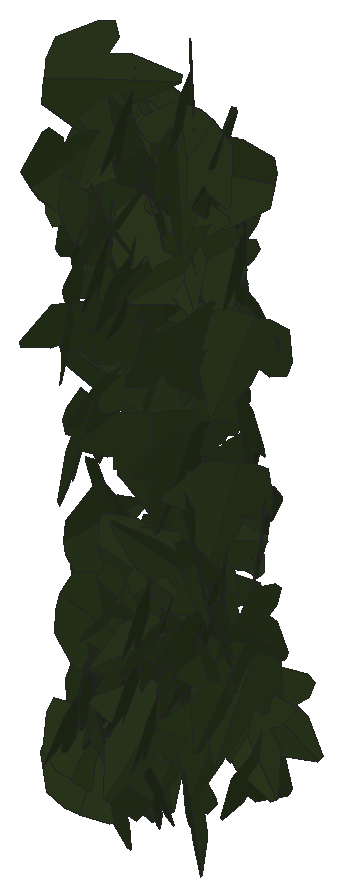
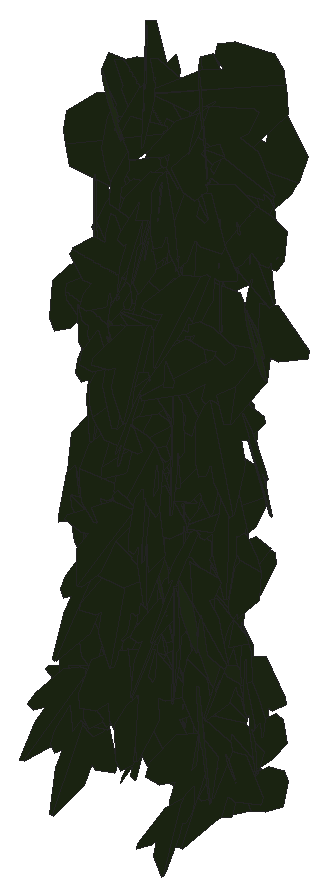
# SketchUp Ruby script. Lengths in inches.
U = 1.inch
M = Sketchup.active_model
def pt(a) = Geom::Point3d.new(a.map { |v| v * U })
def face(e, loops, mat)
  f = e.add_face(loops[0].map { |a| pt(a) })
  loops[1..].each { |l| e.add_face(l.map { |a| pt(a) }).erase! }
  f.material = f.back_material = mat if mat
  f
end
# faces: each face lists its corners as indices into pts; further lists are holes
def faces(e, pts, list, mat = nil) = list.each { |f| face(e, (f[0].is_a?(Array) ? f : [f]).map { |l| l.map { |i| pts[i] } }, mat) }
# xy, xz, yz: faces in a plane at the given z, y or x. An outline is a flat list of corners, or four numbers for a rectangle; further outlines are holes
def ring(l) = l.size == 4 ? [[l[0], l[1]], [l[2], l[1]], [l[2], l[3]], [l[0], l[3]]] : l.each_slice(2).to_a
def flat(e, list, mat, &to3) = list.each { |f| face(e, (f[0].is_a?(Array) ? f : [f]).map { |l| ring(l).map { |u, v| to3.(u, v) } }, mat) }
def xy(e, z, list, mat = nil) = flat(e, list, mat) { |x, y| [x, y, z] }
def xz(e, y, list, mat = nil) = flat(e, list, mat) { |x, z| [x, y, z] }
def yz(e, x, list, mat = nil) = flat(e, list, mat) { |y, z| [x, y, z] }
def lines(e, pts, list) = list.each { |a, b| e.add_line(pt(pts[a]), pt(pts[b])) }
# prism: a flat outline (further loops are holes) pulled along v
def prism(e, loops, v, mat = nil)
  f = face(e, loops, mat); d = Geom::Vector3d.new(v.map { |x| x * U })
  f.pushpull(f.normal.samedirection?(d) ? d.length : -d.length)
end
def box(e, o, s, mat = nil) = prism(e, [[o, [o[0] + s[0], o[1], o[2]], [o[0] + s[0], o[1] + s[1], o[2]], [o[0], o[1] + s[1], o[2]]]], [0, 0, s[2]], mat)
def at(x, y, z, deg = 0) = Geom::Transformation.translation(pt([x, y, z])) * Geom::Transformation.rotation(ORIGIN, Z_AXIS, deg.degrees)
def axes(o, x, y, z) = Geom::Transformation.new([*x, 0, *y, 0, *z, 0, *pt(o).to_a, 1])
def part(name) = M.definitions.add(name)
# library, detail: a bought-in or finely detailed component or shape, given as its bounding box
def library(name, o, s) = part(name).tap { |d| box(d.entities, o, s) }
def detail(e, o, s) = box(e.add_group.entities, o, s)
def put(e, d, t, mat = nil) = e.add_instance(d, t).tap { |i| i.material = mat if mat }
def group(e, t, mat = nil) = e.add_group.tap { |g| g.transformation = t; g.material = mat if mat }.entities
root = M.entities
M.materials.add("efeu2").color = [43, 57, 29]
c1 = part("ivyleaf_10")
p = [[0,0.5,-0.03],[-0.0625,2.02,-0.43],[-0.19,2.01,-0.46],[-0.54,1.05,-0.29],[-0.52,0.625,-0.18],[-0.83,0.76,-0.28],
  [-1.16,0.64,-0.33],[-1.15,0.33,-0.24],[-0.77,-0.39,0.02],[-0.3,-0.51,0.16],[0.04,-0.48,0.23],[-0.02,2.01,-0.4375],
  [-0.06,2.01,-0.43],[0.04,-0.49,0.23],[0.67,-0.49,0.14],[1.38,0.36,-0.2],[1.375,0.51,-0.24],[0.81,0.65,-0.19],
  [0.62,0.59,-0.15],[0.6,1.09,-0.28],[0.5,1.23,-0.31]]
faces(c1.entities,p,[[0,1,2,3,4,5,6,7,8,9,10],[11,12,0,13,14,15,16,17,18,19,20]],"efeu2")
put(root,c1,axes([506.9,136.79,173.25],[0.14298,-0.57574,-0.30284],[-0.08063,0.292,-0.59319],[0.64552,0.164,-0.00701]))
put(root,c1,axes([507.25,136.87,180.96],[-0.48159,0.04123,0.55153],[-0.55018,0.03894,-0.48332],[-0.05645,-0.73116,0.00536]))
put(root,c1,axes([506.58,137.23,179.57],[0.28434,-0.41575,0.47022],[0.3227,-0.34593,-0.501],[0.53835,0.42695,0.05196]))
put(root,c1,axes([506.88,137.7,177.9],[0.03406,-0.68562,-0.00532],[-0.00302,0.00518,-0.68646],[0.68563,0.03408,-0.00276]))
put(root,c1,axes([506.67,137.17,172.16],[0.25361,0.41099,-0.45403],[0.22987,0.38118,0.49226],[0.60538,-0.31691,0.00328]))
put(root,c1,axes([506.84,137.01,177.54],[0.4432,-0.50153,-0.03424],[-0.0221,0.0258,-0.67395],[0.54237,0.41088,0.00052]))
put(root,c1,axes([506.89,137.09,179.24],[-0.46172,-0.52625,-0.10401],[0.07279,0.0745,-0.70007],[0.53147,-0.46739,0.00552]))
put(root,c1,axes([507.1,137.3,176.33],[-0.55796,0.2577,0.27413],[-0.26708,0.07405,-0.61323],[-0.26499,-0.61724,0.04088]))
put(root,c1,axes([506.98,137.88,173.2],[0.21629,-0.56569,-0.2598],[-0.08303,0.24636,-0.60555],[0.61694,0.23148,0.00958]))
put(root,c1,axes([506.71,136.54,181.61],[-0.09839,-0.31052,0.53966],[0.14335,0.5017,0.33646],[-0.63717,0.16082,-0.00764]))
put(root,c1,axes([506.73,137.27,171.58],[0.59865,0.26422,-0.18769],[0.17611,0.07732,0.63862],[0.29733,-0.57779,-0.00037]))
put(root,c1,axes([506.84,138.72,171.91],[-0.02473,0.55753,-0.00621],[0.00369,-0.00584,-0.58031],[-0.60216,-0.02293,-0.0033]))
put(root,c1,axes([506.58,137.39,181.29],[0.5485,0.17555,0.41224],[0.36114,0.21247,-0.571],[-0.2652,0.65242,0.07504]))
put(root,c1,axes([507.17,136.57,180.82],[0.24842,-0.09066,0.51979],[-0.34502,0.40074,0.22851],[-0.42651,-0.37698,0.11791]))
put(root,c1,axes([507.09,136.9375,173.84],[0.05979,-0.2875,-0.63142],[-0.0329,0.63188,-0.29083],[0.69302,0.0548,0.04067]))
put(root,c1,axes([507.38,137.47,182.34],[-0.27318,-0.29829,0.51186],[-0.35183,-0.36898,-0.40669],[0.51239,-0.41239,-0.00635]))
put(root,c1,axes([507.08,137.7,172.24],[-0.609,-0.27487,-0.13611],[0.12561,0.05254,-0.66815],[0.27983,-0.62181,0.00371]))
put(root,c1,axes([507.03,138.19,180.26],[0.03283,0.53443,0.24861],[0.00153,0.2393,-0.55658],[-0.63229,0.02833,0.01156]))
put(root,c1,axes([506.68,137.18,173.43],[0.29168,-0.18018,0.59082],[0.56331,-0.19048,-0.33618],[0.25342,0.63077,0.06725]))
put(root,c1,axes([507.02,137.0625,181.28],[-0.66421,-0.04385,-0.21378],[0.22186,0.009,-0.64121],[0.048,-0.64839,0.00556]))
put(root,c1,axes([507.1,136.64,181.57],[-0.02237,0.43314,0.45119],[-0.07644,0.4295,-0.44947],[-0.65766,-0.06465,0.0369]))
put(root,c1,axes([506.93,137.43,179.04],[0.15008,0.12887,0.69477],[0.1279,0.69359,-0.15627],[-0.69495,0.15547,0.12128]))
put(root,c1,axes([507.14,137.45,174.3125],[0.15323,-0.55835,0.32624],[0.08521,-0.31492,-0.57899],[0.64103,0.17532,-0.00102]))
put(root,c1,axes([507.19,138.24,174.93],[0.32095,-0.51181,-0.2376],[0.00169,0.27421,-0.5884],[0.56427,0.29029,0.13691]))
put(root,c1,axes([507.17,137.69,173.66],[0.08189,-0.52853,0.43053],[0.08188,-0.42286,-0.53469],[0.67675,0.11512,0.0126]))
put(root,c1,axes([507.61,137.62,174.82],[-0.38669,-0.02044,0.48346],[-0.5014,-0.02372,-0.37297],[0.03377,-0.58629,-0.00177]))
put(root,c1,axes([507.36,137.71,180.73],[-0.67386,0.01628,0.13224],[-0.13231,-0.00125,-0.67404],[-0.01573,-0.68671,0.00436]))
put(root,c1,axes([507.31,136.95,180.6],[0.18928,-0.53998,-0.39955],[-0.08333,0.39303,-0.57065],[0.66654,0.20248,0.04212]))
put(root,c1,axes([507.12,137.76,179.85],[-0.53879,-0.3581,-0.20826],[0.22409,0.03542,-0.64065],[0.34841,-0.57655,0.08999]))
put(root,c1,axes([507.17,136.64,176.05],[0.02579,-0.06365,0.59985],[-0.05409,0.57489,0.06813],[-0.62436,-0.05244,0.01887]))
put(root,c1,axes([507.14,136.55,174.95],[-0.00618,0.43263,0.48163],[-0.02651,0.46263,-0.44978],[-0.68393,-0.02184,0.01308]))
put(root,c1,axes([506.82,136.83,183.15],[-0.07026,-0.02384,-0.72695],[0.65355,0.31847,-0.07361],[0.31922,-0.65725,-0.0093]))
put(root,c1,axes([507.53,137.45,174.31],[-0.59782,-0.14347,0.15385],[-0.15413,-0.03901,-0.5947],[0.16057,-0.57163,0.00197]))
put(root,c1,axes([506.89,137.1,175.3125],[-0.09933,0.04464,-0.68674],[0.56951,-0.38419,-0.10734],[-0.38634,-0.57782,0.01832]))
put(root,c1,axes([507.44,137.95,177.9],[0.37613,-0.4555,-0.31889],[-0.04582,0.3583,-0.56583],[0.55414,0.3388,0.16967]))
put(root,c1,axes([507.52,137.35,182.45],[0.38884,0.29811,-0.35452],[-0.28376,-0.21719,-0.48613],[-0.39834,0.44571,0.00023]))
put(root,c1,axes([507.57,137.73,180.09],[-0.439,-0.49286,0.16997],[-0.02017,-0.20599,-0.64937],[0.52095,-0.4233,0.1181]))
put(root,c1,axes([507.375,137.74,174.93],[0.23268,-0.47713,0.31676],[0.15414,-0.26957,-0.54418],[0.59158,0.2579,0.0172]))
put(root,c1,axes([507.43,137.34,180.02],[0.07021,0.57173,0.44951],[-0.03773,0.45386,-0.57136],[-0.7263,0.03168,0.07314]))
put(root,c1,axes([507.09,137.77,178.98],[0.41379,0.00326,-0.54265],[0.50595,0.2444,0.38728],[0.19619,-0.63715,0.14577]))
put(root,c1,axes([507.03,137.42,171.875],[0.10377,-0.08511,-0.7135],[0.54321,-0.46261,0.13418],[-0.47037,-0.55302,-0.00244]))
put(root,c1,axes([507.48,137.55,175.43],[0.11447,-0.4952,-0.43868],[0.13951,0.45325,-0.47525],[0.64668,-0.01013,0.18017]))
put(root,c1,axes([507.71,137.37,172.31],[-0.51777,0.36658,0.27419],[-0.22529,0.1563,-0.6344],[-0.39851,-0.56466,0.0024]))
put(root,c1,axes([507.46,137.57,182.59],[0.09528,0.54935,0.01156],[-0.00154,0.01149,-0.57863],[-0.59341,0.08818,0.00336]))
put(root,c1,axes([507.63,137.33,179.99],[0.18603,-0.63952,-0.18734],[-0.05193,0.17999,-0.66603],[0.66436,0.19314,0.0004]))
put(root,c1,axes([507.41,137.4,177.05],[-0.46287,0.22473,-0.30946],[0.28739,-0.13324,-0.50327],[-0.28212,-0.50445,-0.00494]))
put(root,c1,axes([507.67,137.42,180.86],[-0.21695,-0.64043,-0.11482],[0.06907,0.09768,-0.67535],[0.64697,-0.22518,0.0336]))
put(root,c1,axes([507.66,138.09,174.6],[-0.17825,0.49977,0.26514],[-0.09342,0.2399,-0.54733],[-0.59867,-0.18624,0.00647]))
put(root,c1,axes([508.05,136.78,182.37],[-0.42142,0.09736,0.48472],[-0.50039,0.06123,-0.41672],[-0.11851,-0.60476,0.03584]))
put(root,c1,axes([507.72,136.91,182.95],[0.25353,-0.61713,-0.25077],[-0.04077,0.25344,-0.66492],[0.66488,0.25086,0.05485]))
put(root,c1,axes([507.64,137.68,181.33],[-0.67868,-0.06143,-0.11158],[0.11154,0.00544,-0.68144],[0.0615,-0.68777,0.00458]))
put(root,c1,axes([507.75,137.64,181.38],[0.03236,-0.68955,-0.00584],[-0.00999,0.00537,-0.69024],[0.6895,0.03244,-0.00972]))
put(root,c1,axes([508.13,137.32,181.83],[-0.27876,0.03467,0.53386],[-0.54992,0.06513,-0.27084],[-0.07968,-0.57087,0.00152]))
put(root,c1,axes([507.77,136.92,180.42],[0.02069,-0.57405,-0.40253],[0.01707,0.403,-0.57384],[0.70091,0.00713,0.02586]))
put(root,c1,axes([507.8,137.4375,178.23],[0.40243,0.42699,-0.23491],[-0.24978,-0.09274,-0.57913],[-0.45801,0.42575,0.10944]))
put(root,c1,axes([507.81,137.29,179.79],[-0.18125,-0.6679,0.0763],[-0.00602,-0.07741,-0.6919],[0.67222,-0.18077,0.01438]))
put(root,c1,axes([507.82,136.97,174.01],[0.21995,-0.58813,-0.24273],[-0.04493,0.24183,-0.62666],[0.63467,0.22095,0.03976]))
put(root,c1,axes([507.32,136.96,175.77],[-0.18678,-0.01314,-0.5707],[0.579,-0.12751,-0.17255],[-0.12722,-0.56105,0.05258]))
put(root,c1,axes([507.75,138.41,179.25],[0.11452,0.53998,0.18204],[-0.10046,0.19218,-0.558],[-0.60477,0.07032,0.12716]))
put(root,c1,axes([507.83,138.1,176.28],[0.06611,-0.62024,-0.20868],[0.00551,0.21026,-0.6232],[0.65438,0.0609,0.02633]))
put(root,c1,axes([507.89,138.09,172.87],[-0.22657,-0.5453,0.26649],[0.02259,-0.29184,-0.57795],[0.60651,-0.19284,0.12108]))
put(root,c1,axes([507.91,138.16,180.43],[-0.40528,0.45057,0.0565],[0.03412,-0.04439,0.60982],[0.48896,0.37657,0.00428]))
put(root,c1,axes([507.79,138.54,178.29],[-0.28382,0.49292,-0.09531],[0.04123,-0.08349,-0.58092],[-0.53991,-0.2655,0.00574]))
put(root,c1,axes([508.01,137.24,173.29],[-0.31999,-0.44489,0.41652],[-0.0211,-0.46207,-0.50976],[0.60907,-0.24974,0.20117]))
put(root,c1,axes([508.04,137.07,177.84],[-0.53452,-0.51019,0.01267],[-0.00802,-0.00995,-0.73892],[0.51028,-0.53457,0.00167]))
put(root,c1,axes([508.03,137.46,180.23],[-0.14531,-0.67577,-0.0284],[-0.00877,0.03093,-0.69105],[0.67631,-0.14479,-0.01506]))
put(root,c1,axes([508.01,138.37,179.05],[-0.62141,-0.05793,-0.00008],[0.00008,0.00002,-0.60142],[0.06256,-0.57538,-0.00002]))
put(root,c1,axes([508.03,137.65,178.8125],[0.00198,-0.66951,0.11793],[-0.00178,-0.11793,-0.66951],[0.67981,0.00164,-0.0021]))
put(root,c1,axes([508.33,138.47,178.01],[-0.3906,0.16269,-0.41881],[-0.39216,0.17426,0.41237],[0.25736,0.51245,-0.00727]))
put(root,c1,axes([508.06,137.37,174.52],[0.04649,-0.66784,-0.00346],[0.00151,0.00357,-0.66945],[0.66784,0.04648,0.00175]))
put(root,c1,axes([508.16,138.19,173.53],[-0.5671,-0.28892,0.10619],[-0.08947,-0.05827,-0.63636],[0.29453,-0.574,0.01115]))
put(root,c1,axes([508.09,136.85,175.37],[0.24766,-0.57451,-0.26696],[-0.04468,0.27009,-0.62267],[0.63193,0.24425,0.0606]))
put(root,c1,axes([508.35,137.4,174.69],[-0.17213,-0.19334,0.64929],[-0.32026,-0.56712,-0.25377],[0.59699,-0.35998,0.05108]))
put(root,c1,axes([508.04,136.9,182.07],[-0.51054,0.3714,-0.01802],[0.01708,-0.00793,-0.62521],[-0.40119,-0.47297,-0.00368]))
put(root,c1,axes([508.1,137.57,175.24],[0.33149,-0.57992,-0.07876],[-0.03105,0.07296,-0.66791],[0.58442,0.33281,0.00918]))
put(root,c1,axes([508.19,137.73,176.71],[0.35212,-0.34793,-0.46763],[-0.15254,0.47228,-0.46626],[0.56255,0.34585,0.16627]))
put(root,c1,axes([508.18,136.9,173.58],[0.25052,-0.54009,-0.30576],[-0.07924,0.29919,-0.59342],[0.61555,0.25832,0.04804]))
put(root,c1,axes([508.04,138,177.04],[-0.54715,0.25716,-0.17923],[0.16481,-0.08012,-0.59087],[-0.29089,-0.5291,0.00237]))
put(root,c1,axes([508.28,137.17,174.75],[-0.71609,0.16899,0.1082],[-0.10519,0.02536,-0.73576],[-0.17088,-0.72378,-0.00052]))
put(root,c1,axes([508.33,137.67,178.17],[-0.44863,-0.45978,0.22389],[-0.08489,-0.22675,-0.63575],[0.5043,-0.4472,0.09216]))
put(root,c1,axes([508.49,137.7,180.92],[-0.36034,-0.20672,0.45475],[-0.28398,-0.36832,-0.38976],[0.43842,-0.40848,0.1213]))
put(root,c1,axes([508.52,137.31,175.81],[-0.21656,-0.25046,0.49137],[-0.30624,-0.37802,-0.33356],[0.48965,-0.34719,0.00871]))
put(root,c1,axes([508.38,137.68,180.6],[-0.61618,-0.018,0.0319],[-0.03286,-0.00815,-0.5936],[0.01988,-0.5713,0.00747]))
put(root,c1,axes([507.97,138.33,175.59],[-0.34336,-0.18796,0.45855],[0.43498,0.18207,0.38275],[-0.28064,0.51218,0.03222]))
put(root,c1,axes([508.39,137.66,180.74],[-0.22177,0.44283,0.2844],[-0.15177,0.23588,-0.50699],[-0.54122,-0.2476,0.02564]))
put(root,c1,axes([508.36,138.33,180.18],[0.09998,-0.37086,0.42469],[-0.11486,0.3943,0.39749],[-0.58458,-0.1409,-0.00547]))
put(root,c1,axes([508.15,138.33,176.08],[0.2586,0.41965,0.31362],[0.14707,0.26937,-0.50231],[-0.53838,0.27516,0.01343]))
put(root,c1,axes([508.84,137.06,175.67],[-0.38001,0.08081,-0.59231],[-0.59775,-0.06087,0.37519],[-0.0081,0.7011,0.10085]))
put(root,c1,axes([508.4,138.01,174.79],[0.06023,0.53339,0.18628],[-0.15211,0.1875,-0.53508],[-0.58833,0.00613,0.15741]))
put(root,c1,axes([508.1,137.15,181.21],[0.56572,0.29753,0.29738],[0.26396,0.13697,-0.63919],[-0.32754,0.62427,-0.00149]))
put(root,c1,axes([508.1875,137.6,177.21],[0.2261,0.13706,0.51488],[0.18153,0.4869,-0.21412],[-0.52425,0.22771,0.14792]))
put(root,c1,axes([508.34,137.73,174.02],[-0.53623,0.23221,-0.15333],[0.1404,-0.07001,-0.56999],[-0.26179,-0.51319,0.00837]))
put(root,c1,axes([508.54,137.46,174.59],[-0.03505,-0.6328,0.20775],[-0.02677,-0.20653,-0.6336],[0.66549,-0.04163,-0.01455]))
put(root,c1,axes([508.51,137.25,183.43],[0.27814,-0.56193,-0.33488],[-0.03249,0.35157,-0.61694],[0.65334,0.25671,0.11188]))
put(root,c1,axes([508.51,137.19,177.7],[0.01936,-0.6638,0.17093],[0.02701,-0.17013,-0.66374],[0.68492,0.02547,0.02134]))
put(root,c1,axes([508.54,137.96,179.16],[-0.13125,0.29275,0.47489],[0.05257,-0.46017,0.3203],[0.58344,0.10732,0.07797]))
put(root,c1,axes([508.8125,137.44,180.67],[0.22535,0.212,-0.55535],[-0.47616,-0.3052,-0.30518],[-0.39787,0.48533,0.05068]))
put(root,c1,axes([508.75,137.75,179.29],[-0.37185,-0.4442,0.26105],[-0.15172,-0.20857,-0.58427],[0.52973,-0.37155,0.0159]))
put(root,c1,axes([508.46,137.43,172.125],[-0.17827,0.49763,-0.19913],[0.07875,-0.17749,-0.54511],[-0.57044,-0.18002,-0.01302]))
put(root,c1,axes([508.3125,138.17,178.56],[0.32021,-0.38332,-0.3323],[0.2163,-0.24901,0.50396],[-0.49364,-0.35776,0.00527]))
put(root,c1,axes([508.66,137.84,173.21],[-0.21933,-0.57746,0.25104],[0.0166,-0.27104,-0.60897],[0.62944,-0.19407,0.10354]))
put(root,c1,axes([508.52,138.57,176.89],[0.07475,-0.29579,0.48741],[0.20651,-0.43056,-0.31198],[0.56179,0.19763,0.04983]))
put(root,c1,axes([508.6875,136.97,179.63],[-0.26214,-0.60669,-0.21946],[0.06746,0.20981,-0.66059],[0.64163,-0.26993,-0.02021]))
put(root,c1,axes([508.2,138.04,175.73],[0.19752,-0.04318,-0.54411],[0.54247,-0.14668,0.19519],[-0.16483,-0.53447,-0.00961]))
put(root,c1,axes([508.83,137.08,182.71],[0.64722,-0.06851,-0.29641],[-0.29362,0.04167,-0.65076],[0.07962,0.71064,0.00958]))
put(root,c1,axes([508.6,137.98,181.69],[-0.03576,-0.04442,-0.6253],[0.04206,-0.60106,0.04395],[-0.64976,-0.03647,0.03726]))
put(root,c1,axes([508.67,136.9,182.52],[-0.01238,0.64743,-0.11662],[-0.02558,-0.11248,-0.67292],[-0.70917,-0.00724,0.02631]))
put(root,c1,axes([508.83,137.17,175.03],[0.04766,-0.68054,-0.00545],[-0.00155,0.00536,-0.68221],[0.68056,0.04767,-0.00117]))
put(root,c1,axes([509.22,137.81,181.88],[-0.08706,-0.02791,-0.59547],[-0.58428,-0.1875,0.08872],[-0.20473,0.54697,0.00003]))
put(root,c1,axes([508.91,138.28,172.37],[-0.07824,-0.49117,-0.42011],[0.06691,0.41475,-0.49736],[0.64285,-0.10295,0.00063]))
put(root,c1,axes([508.95,138,173.875],[-0.26418,-0.54315,0.26373],[0.05507,-0.30834,-0.57987],[0.60128,-0.2104,0.16898]))
put(root,c1,axes([508.97,137.65,177.05],[-0.31008,-0.57285,0.18808],[0.031,-0.22636,-0.63834],[0.60214,-0.28334,0.12971]))
put(root,c1,axes([509,137.84,178.28],[-0.49544,0.36208,0.10576],[-0.1283,0.01268,-0.60429],[-0.38538,-0.46971,0.06521]))
put(root,c1,axes([508.44,137.17,176.46],[0.3614,-0.22205,0.61466],[0.59408,-0.18109,-0.41472],[0.27236,0.68965,0.089]))
put(root,c1,axes([508.96,137.72,174.18],[-0.08942,-0.59036,0.31044],[0.03831,-0.31724,-0.59226],[0.6659,-0.06102,0.07576]))
put(root,c1,axes([508.48,138.42,179.46],[0.01377,-0.06911,0.57845],[0.58978,-0.1237,-0.029],[0.13625,0.54242,0.06709]))
put(root,c1,axes([508.58,138.2,173.04],[0.48635,0.23696,0.35419],[0.3257,0.13991,-0.54082],[-0.27482,0.58517,-0.01412]))
put(root,c1,axes([509,137.37,175.76],[0.25274,-0.58427,-0.23219],[-0.04831,0.23146,-0.63502],[0.62686,0.2534,0.04467]))
put(root,c1,axes([509.16,138.18,176.3],[-0.22957,0.51328,0.12421],[-0.26892,0.01568,-0.53097],[-0.50161,-0.24332,0.22781]))
put(root,c1,axes([509.01,137.9,174.7],[-0.07092,-0.46994,-0.45003],[0.11649,0.43622,-0.47387],[0.64016,-0.13144,0.03637]))
put(root,c1,axes([508.85,138.52,173.15],[-0.17189,-0.49294,-0.36364],[0.33354,0.24147,-0.48499],[0.51378,-0.32167,0.19319]))
put(root,c1,axes([509,137.52,182.7],[0.30872,-0.49297,0.14562],[0.08416,-0.11665,-0.59258],[0.54703,0.29616,0.00898]))
put(root,c1,axes([509.18,137.08,175.32],[-0.31704,0.3568,0.33082],[-0.21585,0.24748,-0.48051],[-0.46896,-0.35512,-0.00248]))
put(root,c1,axes([509.21,137.7,179.47],[-0.46713,-0.42349,0.25015],[-0.09635,-0.25952,-0.61928],[0.48233,-0.46199,0.11857]))
put(root,c1,axes([509.1,137.71,180.91],[0.30306,-0.56381,-0.24768],[-0.00563,0.2735,-0.62948],[0.61579,0.27998,0.11614]))
